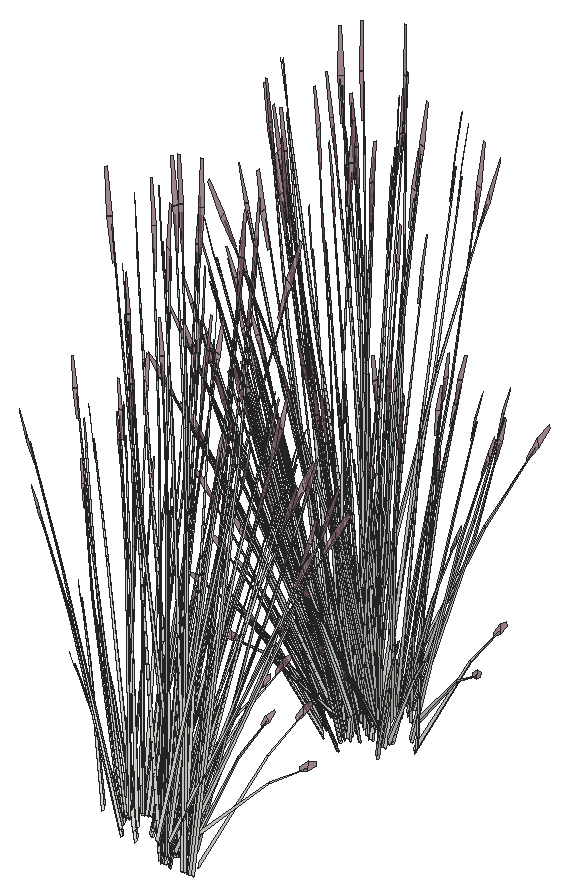
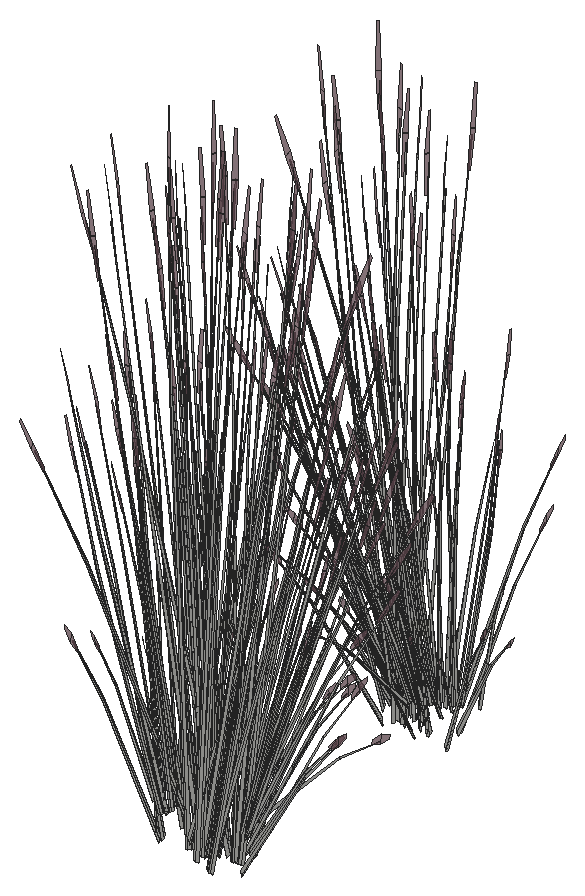
# SketchUp Ruby script. Lengths in inches.
U = 1.inch
M = Sketchup.active_model
def pt(a) = Geom::Point3d.new(a.map { |v| v * U })
def face(e, loops, mat)
  f = e.add_face(loops[0].map { |a| pt(a) })
  loops[1..].each { |l| e.add_face(l.map { |a| pt(a) }).erase! }
  f.material = f.back_material = mat if mat
  f
end
# faces: each face lists its corners as indices into pts; further lists are holes
def faces(e, pts, list, mat = nil) = list.each { |f| face(e, (f[0].is_a?(Array) ? f : [f]).map { |l| l.map { |i| pts[i] } }, mat) }
# xy, xz, yz: faces in a plane at the given z, y or x. An outline is a flat list of corners, or four numbers for a rectangle; further outlines are holes
def ring(l) = l.size == 4 ? [[l[0], l[1]], [l[2], l[1]], [l[2], l[3]], [l[0], l[3]]] : l.each_slice(2).to_a
def flat(e, list, mat, &to3) = list.each { |f| face(e, (f[0].is_a?(Array) ? f : [f]).map { |l| ring(l).map { |u, v| to3.(u, v) } }, mat) }
def xy(e, z, list, mat = nil) = flat(e, list, mat) { |x, y| [x, y, z] }
def xz(e, y, list, mat = nil) = flat(e, list, mat) { |x, z| [x, y, z] }
def yz(e, x, list, mat = nil) = flat(e, list, mat) { |y, z| [x, y, z] }
def lines(e, pts, list) = list.each { |a, b| e.add_line(pt(pts[a]), pt(pts[b])) }
# prism: a flat outline (further loops are holes) pulled along v
def prism(e, loops, v, mat = nil)
  f = face(e, loops, mat); d = Geom::Vector3d.new(v.map { |x| x * U })
  f.pushpull(f.normal.samedirection?(d) ? d.length : -d.length)
end
def box(e, o, s, mat = nil) = prism(e, [[o, [o[0] + s[0], o[1], o[2]], [o[0] + s[0], o[1] + s[1], o[2]], [o[0], o[1] + s[1], o[2]]]], [0, 0, s[2]], mat)
def at(x, y, z, deg = 0) = Geom::Transformation.translation(pt([x, y, z])) * Geom::Transformation.rotation(ORIGIN, Z_AXIS, deg.degrees)
def axes(o, x, y, z) = Geom::Transformation.new([*x, 0, *y, 0, *z, 0, *pt(o).to_a, 1])
def part(name) = M.definitions.add(name)
# library, detail: a bought-in or finely detailed component or shape, given as its bounding box
def library(name, o, s) = part(name).tap { |d| box(d.entities, o, s) }
def detail(e, o, s) = box(e.add_group.entities, o, s)
def put(e, d, t, mat = nil) = e.add_instance(d, t).tap { |i| i.material = mat if mat }
def group(e, t, mat = nil) = e.add_group.tap { |g| g.transformation = t; g.material = mat if mat }.entities
root = M.entities
M.materials.add("LightPink_Translucent").color = [144, 107, 117]
M.materials["LightPink_Translucent"].alpha = 0.75
c1 = part("blade")
p = [[2.15,0.21,22],[0,0.17,0],[0.09,0.45,0],[2.18,0.31,22],[2.29,0.31,22],[0.38,0.45,0],
  [2.48,0.24,33],[2.49,0.24,33],[2.48,0.22,33]]
faces(c1.entities,p,[[0,1,2,3],[4,5,2,3],[6,3,4,7],[8,0,3,6]])
c2 = part("seeds")
p = [[0.3,-0.1,1.38],[-0.01,-0.03,1.59],[-0.01,-0.03,0.03],[0.14,-0.07,-0.07],[0.29,-0.03,3],[0.15,0.01,3.11]]
faces(c2.entities,p,[[0,1,2,3],[1,0,4,5]],"LightPink_Translucent")
c3 = part("blade with seeds")
put(c3.entities,c1,at(0,0,0))
put(c3.entities,c2,axes([2.4,0.25,30.99],[1.5799,-0.05474,1.17369],[-0.12525,1.92788,0.29478],[-0.07173,-0.02425,1.56792]))
put(root,c3,axes([359.76,228.125,201.54],[0.11943,-0.00833,1.31208],[0.32759,-0.38275,-0.2075],[0.21244,0.05052,0.10523]))
put(root,c3,axes([358.36,228.87,199.64],[-0.34375,-0.4954,-0.03857],[0.58235,-0.27531,0.38706],[-0.1435,0.04717,1.22723]))
put(root,c3,axes([358.24,227.67,199.96],[0.41131,0.296,0.1086],[-0.34309,0.33395,-0.3101],[-0.0955,0.04515,0.95058]))
put(root,c3,axes([354.99,227.75,201.55],[-0.13808,-0.45342,0.36002],[0.54163,-0.07869,0.29685],[-0.15963,0.10664,0.74497]))
put(root,c3,axes([354.88,227.66,201.55],[-0.3822,-0.20719,0.04823],[0.22252,-0.29505,0.37966],[-0.12254,0.09539,0.57892]))
put(root,c3,axes([355.06,227.12,200.91],[0.19317,-0.10421,1.28532],[0.16263,0.48153,0.10393],[-0.30326,0.10883,0.54946]))
put(root,c3,axes([359.3,228.1875,201.74],[0.55654,0.01186,-0.53284],[-0.03738,0.49951,0.0643],[0.23578,0.05271,0.75375]))
put(root,c3,axes([358.67,228.59,199.86],[0.52105,-0.24633,0.37238],[0.31144,0.44171,0],[-0.11867,0.0561,1.18128]))
put(root,c3,axes([357.93,228.2,199.72],[0.24206,0.56598,-0.04509],[-0.69162,0.19832,0],[0.00845,0.01976,1.2913]))
put(root,c3,axes([358.2,228.81,199.52],[-0.51941,-0.1219,-0.23233],[0.13078,-0.42928,0.23233],[-0.10471,0.0495,1.0423]))
put(root,c3,axes([354.45,227.9375,199.94],[0.19348,0.04044,1.07251],[0.1247,0.41309,-0.23066],[-0.26282,0.07733,0.45856]))
put(root,c3,axes([355.32,227.6,201.79],[0.48462,-0.07041,0.2656],[0.12797,0.4025,-0.3429],[-0.13888,0.10811,0.65611]))
put(root,c3,axes([360.21,227.17,199.78],[0.69617,0,0],[0,0.55062,-0.38706],[0,0.12541,1.22783]))
put(root,c3,axes([353.46,227.42,201.53],[0.07105,0.01321,1.33037],[0.2198,0.43529,-0.12571],[-0.14545,0.11425,0.23543]))
put(root,c3,axes([359.93,227.46,199.65],[-0.69582,-0.00394,-0.03732],[0,-0.55062,0.37457],[-0.02187,0.12535,1.18764]))
put(root,c3,axes([358.43,226.98,200],[0.62699,0.23507,-0.21822],[-0.3019,0.49615,-0.37502],[0.0197,0.12182,1.19781]))
put(root,c3,axes([354.05,228.8,200.07],[0.23202,-0.22328,0.86145],[0.09155,0.35348,0.63294],[-0.16768,0.06329,0.18974]))
put(root,c3,axes([359.64,228.39,201.39],[0.31678,0.30846,-0.2656],[-0.36171,0.29199,0.3429],[0.18378,0.04443,0.65611]))
put(root,c3,axes([359.79,227.54,199.52],[-0.38863,0.30738,-0.23233],[-0.38863,-0.30738,0.23233],[0,0.09901,1.0423]))
put(root,c3,axes([358.11,227.57,200],[0.06488,0.56215,-0.21822],[-0.6757,0.03399,-0.37502],[-0.11898,0.07488,1.19781]))
put(root,c3,axes([359.47,228.51,201.55],[-0.02803,0.37463,0.04823],[-0.42332,-0.01027,0.37966],[0.16216,0.0392,0.57892]))
put(root,c3,axes([358.36,227.35,199.66],[-0.27012,0.44393,-0.33554],[-0.56127,-0.21365,0.16149],[0,0.10233,1.07733]))
put(root,c3,axes([354.93,227.84,201.39],[-0.48462,0.07041,-0.2656],[-0.12797,-0.4025,0.3429],[-0.13888,0.10811,0.65611]))
put(root,c3,axes([359.51,228.39,201.55],[-0.41051,0.32462,0.36002],[-0.35404,-0.34474,0.29685],[0.1926,0.05988,0.74497]))
put(root,c3,axes([354.22,228.74,202.23],[0.49129,0.13151,-0.04866],[-0.15113,0.40475,-0.22062],[-0.08035,0.06145,0.72768]))
put(root,c3,axes([357.71,227.99,199.54],[-0.375,0.3703,-0.46765],[-0.46584,-0.33578,-0.12274],[-0.15027,0.09237,1.03225]))
put(root,c3,axes([358.21,228.77,201.79],[-0.08599,-0.39682,0.2656],[0.49155,-0.10478,-0.3429],[0.13203,0.11372,0.65611]))
put(root,c3,axes([358.375,228.62,199.75],[0.697,0.16013,0.23067],[-0.17437,0.57237,-0.27369],[-0.11536,0.07164,1.23664]))
put(root,c3,axes([358.32,229,199.51],[-0.52105,0.24633,-0.37238],[-0.31144,-0.44171,0],[-0.11867,0.0561,1.18128]))
put(root,c3,axes([360.06,227.55,199.51],[0,0.49266,-0.37238],[-0.62289,0,0],[0,0.11221,1.18128]))
put(root,c3,axes([358.5,227.6,200.91],[-0.2068,-0.08488,1.28532],[0.42797,-0.35609,0.10393],[0.26673,0.16064,0.54946]))
put(root,c3,axes([358.54,226.48,201.36],[-0.48108,-0.25598,1.03712],[0.50798,-0.39855,0.44749],[0.15521,0.24018,1.00248]))
put(root,c3,axes([355.07,227.5625,201.78],[0.515,0.27165,-0.0912],[-0.2967,0.3934,-0.50621],[-0.1455,0.13675,0.76918]))
put(root,c3,axes([359.26,228.57,200.07],[-0.31347,-0.14166,0.86145],[0.40476,-0.14393,0.63294],[0.10917,0.12192,0.18974]))
put(root,c3,axes([358.16,228.97,201.78],[0.33176,-0.4217,-0.0912],[0.48044,0.24295,-0.50621],[0.16701,0.11914,0.76918]))
put(root,c3,axes([355.76,227.44,200.91],[0.13906,-0.15138,1.28532],[0.35111,0.40859,0.10393],[-0.24082,0.18608,0.54946]))
put(root,c3,axes([355.33,227.89,201.51],[0.14302,0.44985,-0.38324],[-0.54163,0.07869,-0.29685],[-0.15522,0.12083,0.7333]))
put(root,c3,axes([355.98,228.4,201.79],[0.3767,-0.25939,0.2656],[0.3566,0.29618,-0.3429],[-0.05426,0.15048,0.65611]))
put(root,c3,axes([358.8,228.93,199.78],[0.34808,0.49367,0],[-0.58235,0.27531,-0.38706],[-0.13264,0.0627,1.22783]))
put(root,c3,axes([357.73,229.32,201.53],[0.00165,-0.05965,1.33037],[0.47711,-0.26315,-0.12571],[0.16572,0.09393,0.23543]))
put(root,c3,axes([359.35,229.09,199.12],[0.04056,-0.07113,1.32257],[0.51066,-0.20948,-0.20205],[0.15482,0.10842,0.22528]))
put(root,c3,axes([358.5,226.97,200.13],[-0.01521,-0.46386,1.05954],[0.68831,0.12024,0.44862],[-0.1628,0.25382,1.00012]))
put(root,c3,axes([358.68,227.48,199.57],[0.20414,0.45107,-0.51909],[-0.58805,0.16245,-0.13624],[0.02256,0.15274,1.1458]))
put(root,c3,axes([355.63,228.64,201.55],[-0.45752,-0.02296,0.04823],[0.01254,-0.34663,0.37966],[-0.04787,0.13278,0.57892]))
put(root,c3,axes([354.66,229.03,199.12],[0.07468,0.04922,1.32257],[0.12663,0.45605,-0.20205],[-0.16551,0.09725,0.22528]))
put(root,c3,axes([355.78,228.67,201.55],[-0.39645,-0.33614,0.36002],[0.42102,-0.2899,0.29685],[-0.07313,0.15771,0.74497]))
put(root,c3,axes([358.56,228.76,201.51],[0.54938,-0.11711,-0.38324],[0.0961,0.44351,-0.29685],[0.14756,0.1271,0.7333]))
put(root,c3,axes([357.03,228.83,201.79],[0.16784,-0.37886,0.2656],[0.48968,0.1105,-0.3429],[0.0449,0.15254,0.65611]))
put(root,c3,axes([359.3125,229.21,200],[-0.35702,-0.01545,0.78795],[0.23577,-0.32816,0.43504],[0.14104,0.11659,0.61808]))
put(root,c3,axes([358.29,229.125,201.55],[-0.25304,0.31296,0.04823],[-0.36033,-0.18221,0.37966],[0.11649,0.10034,0.57892]))
put(root,c3,axes([357.69,230.18,202.23],[0.38473,-0.28263,-0.04866],[0.35252,0.30954,-0.22062],[0.02482,0.08771,0.72768]))
put(root,c3,axes([358.39,229.04,201.55],[-0.55374,0.11306,0.36002],[-0.0961,-0.44351,0.29685],[0.13023,0.13071,0.74497]))
put(root,c3,axes([355.66,227.82,200.91],[0.10366,-0.16934,1.28532],[0.43488,0.35044,0.10393],[-0.19618,0.21841,0.54946]))
put(root,c3,axes([358.15,228.42,199.94],[0.00982,-0.16331,1.07251],[0.4695,-0.18242,-0.23066],[0.14493,0.19547,0.45856]))
put(root,c3,axes([356.88,229.17,201.55],[-0.41024,0.16744,0.04823],[-0.2008,-0.30532,0.37966],[0.03962,0.13459,0.57892]))
put(root,c3,axes([355.78,228.77,201.39],[-0.3767,0.25939,-0.2656],[-0.3566,-0.29618,0.3429],[-0.05426,0.15048,0.65611]))
put(root,c3,axes([354.48,228.69,201.54],[-0.01384,0.09749,1.31208],[0.39274,0.33916,-0.2075],[-0.10282,0.16039,0.10523]))
put(root,c3,axes([355.74,228.47,202.05],[0.61188,0.02441,-0.10123],[-0.01672,0.46217,-0.56189],[-0.0425,0.178,0.85379]))
put(root,c3,axes([356.87,228.99,201.78],[0.54481,-0.22937,-0.0912],[0.26773,0.4071,-0.50621],[0.07188,0.17155,0.76918]))
put(root,c3,axes([357.03,229.14,201.8],[-0.54859,-0.1288,0.39962],[0.18759,-0.42344,0.32951],[0.03297,0.16652,0.82692]))
put(root,c3,axes([356.02,229.78,200.07],[-0.01441,-0.29294,0.86145],[0.36003,0.20894,0.63294],[-0.07081,0.13963,0.18974]))
put(root,c3,axes([356.97,229.08,199.12],[0.0901,-0.02681,1.32257],[0.54199,0.14755,-0.20205],[0.01585,0.1663,0.22528]))
put(root,c3,axes([356.15,228.65,201.75],[0.39855,0.33102,-0.4254],[-0.42102,0.2899,-0.32951],[-0.06064,0.16819,0.81396]))
put(root,c3,axes([355.72,229.15,200.12],[0.50577,-0.08724,0.04881],[0.11627,0.35148,-0.64728],[-0.03206,0.17792,0.5802]))
put(root,c3,axes([357.34,228.97,201.51],[0.54728,0.1235,-0.38324],[-0.18759,0.42344,-0.29685],[0.05018,0.17048,0.7333]))
put(root,c3,axes([357.65,228.1,200.91],[-0.12726,-0.15818,1.28532],[0.58807,-0.13317,0.10393],[0.13291,0.24832,0.54946]))
put(root,c3,axes([357.09,229.23,201.39],[-0.16784,0.37886,-0.2656],[-0.48968,-0.1105,0.3429],[0.0449,0.15254,0.65611]))
put(root,c3,axes([356.03,228.5,202],[-0.01449,0.45571,-0.59145],[-0.61002,-0.03061,0.07138],[-0.06438,0.19306,0.83667]))
put(root,c3,axes([354.4375,229.69,201.53],[0.06316,-0.02974,1.33037],[0.52204,0.19785,-0.12571],[-0.01227,0.16473,0.23543]))
put(root,c3,axes([356.61,228.17,200.91],[-0.01363,-0.18909,1.28532],[0.5906,0.12544,0.10393],[-0.03653,0.26947,0.54946]))
put(root,c3,axes([357.14,228.89,201.74],[0.26572,0.40059,-0.53284],[-0.54698,0.22325,0.0643],[0.06214,0.19355,0.75375]))
put(root,c3,axes([355.6,229.52,199.94],[0.17569,-0.07772,1.07251],[0.43377,0.23434,-0.23066],[-0.12911,0.20277,0.45856]))
put(root,c3,axes([356.74,229.9,201.54],[0.07057,0.07933,1.31208],[0.56952,0.03117,-0.2075],[0.05727,0.17496,0.10523]))
put(root,c3,axes([355.83,229.14,200.52],[0.01223,-0.25433,1.15759],[0.55017,0.13434,0.15997],[-0.04767,0.27105,0.54661]))
put(root,c3,axes([356.25,245.91,200.91],[0.12726,0.15818,1.28532],[-0.58807,0.13317,0.10393],[-0.13291,-0.24832,0.54946]))
put(root,c3,axes([357.22,244.86,201.54],[-0.08515,-0.06907,1.31208],[-0.56828,0.04379,-0.2075],[-0.0907,-0.16522,0.10523]))
put(root,c3,axes([358.54,245.68,199.94],[-0.15825,0.09972,1.07251],[-0.47395,-0.17454,-0.23066],[0.08785,-0.21706,0.45856]))
put(root,c3,axes([357.82,246.03,201.74],[-0.26572,-0.40059,-0.53284],[0.54698,-0.22325,0.0643],[-0.06214,-0.19355,0.75375]))
put(root,c3,axes([356.09,245.49,199.94],[-0.03371,0.16116,1.07251],[-0.49286,0.13491,-0.23066],[-0.11521,-0.20831,0.45856]))
put(root,c3,axes([357.36,245.14,199.12],[-0.09338,0.01775,1.32257],[-0.51641,-0.1998,-0.20205],[0.00867,-0.16666,0.22528]))
put(root,c3,axes([358.92,246.42,201.74],[0.01449,-0.45571,-0.53284],[0.61002,0.03061,0.0643],[0.06438,-0.19306,0.75375]))
put(root,c3,axes([359.77,245.71,201.54],[-0.00537,-0.09805,1.31208],[-0.45391,-0.28338,-0.2075],[0.07018,-0.17178,0.10523]))
put(root,c3,axes([357.87,245.69,201.39],[0.16784,-0.37886,-0.2656],[0.48968,0.1105,0.3429],[-0.0449,-0.15254,0.65611]))
put(root,c3,axes([358.24,246.19,200.91],[-0.10366,0.16934,1.28532],[-0.43488,-0.35044,0.10393],[0.19618,-0.21841,0.54946]))
put(root,c3,axes([359.65,245.36,201.53],[-0.05654,0.03763,1.33037],[-0.55396,-0.12696,-0.12571],[-0.02005,-0.16422,0.23543]))
put(root,c3,axes([357.62,245.95,201.51],[-0.54728,-0.1235,-0.38324],[0.18759,-0.42344,-0.29685],[-0.05018,-0.17048,0.7333]))
put(root,c3,axes([357.95,244.89,200.07],[0.07142,0.28728,0.86145],[-0.3962,-0.15911,0.63294],[0.04263,-0.1471,0.18974]))
put(root,c3,axes([358.8,246.27,201.51],[-0.39855,-0.33102,-0.38324],[0.42102,-0.2899,-0.29685],[0.06064,-0.16819,0.7333]))
put(root,c3,axes([356.64,244.64,201.53],[-0.01039,0.05905,1.33037],[-0.51226,0.21431,-0.12571],[-0.15074,-0.10955,0.23543]))
put(root,c3,axes([356.52,245.69,201.82],[0.62019,-0.12663,0.40322],[0.10763,0.49673,0.33247],[-0.14586,-0.1464,0.83437]))
put(root,c3,axes([357.93,245.78,201.55],[0.54859,0.1288,0.36002],[-0.18759,0.42344,0.29685],[-0.03297,-0.16652,0.74497]))
put(root,c3,axes([358.08,245.93,201.78],[-0.54481,0.22937,-0.0912],[-0.26773,-0.4071,-0.50621],[-0.07188,-0.17155,0.76918]))
put(root,c3,axes([359.22,246.44,201.78],[-0.61188,-0.02441,-0.0912],[0.01672,-0.46217,-0.50621],[0.0425,-0.178,0.76918]))
put(root,c3,axes([359.17,246.15,201.39],[0.3767,-0.25939,-0.2656],[0.3566,0.29618,0.3429],[0.05426,-0.15048,0.65611]))
put(root,c3,axes([355.92,245.23,200.07],[0.29042,0.17147,0.86145],[-0.42295,0.10307,0.63294],[-0.0905,-0.13178,0.18974]))
put(root,c3,axes([358.07,245.75,201.55],[0.41024,-0.16744,0.04823],[0.2008,0.30532,0.37966],[-0.03962,-0.13459,0.57892]))
put(root,c3,axes([356.62,246.14,201.74],[-0.47473,-0.23813,-0.53284],[0.33738,-0.41728,0.0643],[-0.172,-0.14218,0.75375]))
put(root,c3,axes([356.45,245.83,201.39],[-0.08599,-0.39682,-0.2656],[0.49155,-0.10478,0.3429],[-0.13203,-0.11372,0.65611]))
put(root,c3,axes([356.67,245.79,201.55],[0.25304,-0.31296,0.04823],[0.36033,0.18221,0.37966],[-0.11649,-0.10034,0.57892]))
put(root,c3,axes([355.6875,245.75,199.12],[-0.05393,0.0649,1.32257],[-0.545,0.13993,-0.20205],[-0.13166,-0.12729,0.22528]))
put(root,c3,axes([356.59,247.54,199.57],[-0.22864,-0.5052,-0.52377],[0.65862,-0.18195,-0.13747],[-0.02527,-0.17107,1.15612]))
put(root,c3,axes([355.4,246.41,200.91],[0.2068,0.08488,1.28532],[-0.42797,0.35609,0.10393],[-0.26673,-0.16064,0.54946]))
put(root,c3,axes([359.64,245.99,199.12],[-0.08333,-0.03881,1.32257],[-0.21404,-0.4336,-0.20205],[0.14439,-0.11767,0.22528]))
put(root,c3,axes([357.92,246.09,201.79],[-0.16784,0.37886,0.2656],[-0.48968,-0.1105,-0.3429],[-0.0449,-0.15254,0.65611]))
put(root,c3,axes([356.4,246.16,201.51],[-0.54938,0.11711,-0.38324],[-0.0961,-0.44351,-0.29685],[-0.14756,-0.1271,0.7333]))
put(root,c3,axes([359.17,246.25,201.55],[0.39645,0.33614,0.36002],[-0.42102,0.2899,0.29685],[0.07313,-0.15771,0.74497]))
put(root,c3,axes([356.78,245.76,202.07],[-0.37157,0.4723,-0.10215],[-0.5381,-0.2721,-0.56695],[-0.18705,-0.13344,0.86148]))
put(root,c3,axes([359.32,246.28,201.55],[0.45752,0.02296,0.04823],[-0.01254,0.34663,0.37966],[0.04787,-0.13278,0.57892]))
put(root,c3,axes([358.98,246.52,201.79],[-0.3767,0.25939,0.2656],[-0.3566,-0.29618,-0.3429],[0.05426,-0.15048,0.65611]))
put(root,c3,axes([359.64,247.21,201.74],[0.29081,-0.38873,-0.53284],[0.5096,0.27626,0.0643],[0.17364,-0.14084,0.75375]))
put(root,c3,axes([356.5,246.08,199.78],[-0.34808,-0.49367,0],[0.58235,-0.27531,-0.38706],[0.13264,-0.0627,1.22783]))
put(root,c3,axes([359.625,247.03,201.51],[-0.14302,-0.44985,-0.38324],[0.54163,-0.07869,-0.29685],[0.15522,-0.12083,0.7333]))
put(root,c3,axes([357.26,245.49,199.6],[-0.38473,0.28263,-0.02919],[-0.35252,-0.30954,-0.13237],[-0.02482,-0.08771,0.43661]))
put(root,c3,axes([355.36,245.625,201.54],[-0.11979,-0.00348,1.31208],[-0.38137,0.34775,-0.2075],[-0.20349,-0.07106,0.10523]))
put(root,c3,axes([359.88,247.35,201.78],[-0.515,-0.27165,-0.0912],[0.2967,-0.3934,-0.50621],[0.1455,-0.13675,0.76918]))
put(root,c3,axes([357.75,248.84,200.49],[0.48111,0.19866,1.13446],[-0.47133,0.42798,0.44862],[-0.21112,-0.25366,0.95105]))
put(root,c3,axes([356.75,246.15,201.79],[0.08599,0.39682,0.2656],[-0.49155,0.10478,-0.3429],[-0.13203,-0.11372,0.65611]))
put(root,c3,axes([355.24,247.46,199.51],[0,-0.49266,-0.37238],[0.62289,0,0],[0,-0.11221,1.18128]))
put(root,c3,axes([356.97,246.01,199.51],[0.52105,-0.24633,-0.37238],[0.31144,0.44171,0],[0.11867,-0.0561,1.18128]))
put(root,c3,axes([360.0625,246.86,199.94],[-0.19889,-0.01459,1.07251],[-0.20376,-0.39145,-0.23066],[0.24434,-0.11074,0.45856]))
put(root,c3,axes([355.27,246.41,201.82],[0.45978,-0.36358,0.40322],[0.39653,0.38611,0.33247],[-0.21571,-0.06707,0.83437]))
put(root,c3,axes([361.15,247.24,201.53],[-0.07272,-0.00374,1.33037],[-0.30197,-0.40092,-0.12571],[0.12127,-0.13182,0.23543]))
put(root,c3,axes([357.59,247.02,199.54],[0.375,-0.3703,-0.46765],[0.46584,0.33578,-0.12274],[0.15027,-0.09237,1.03225]))
put(root,c3,axes([360.29,246.14,200.07],[-0.18544,0.25079,0.86145],[-0.15939,-0.33694,0.63294],[0.15316,-0.08443,0.18974]))
put(root,c3,axes([360.03,247.08,201.39],[0.48462,-0.07041,-0.2656],[0.12797,0.4025,0.3429],[0.13888,-0.10811,0.65611]))
put(root,c3,axes([355.48,246.41,201.55],[0.02803,-0.37463,0.04823],[0.42332,0.01027,0.37966],[-0.16216,-0.0392,0.57892]))
put(root,c3,axes([356.93,247.67,199.66],[0.27012,-0.44393,-0.33554],[0.56127,0.21365,0.16149],[0,-0.10233,1.07733]))
put(root,c3,axes([355.32,246.53,201.39],[-0.31678,-0.30846,-0.2656],[0.36171,-0.29199,0.3429],[-0.18378,-0.04443,0.65611]))
put(root,c3,axes([357.18,247.45,200],[-0.06488,-0.56215,-0.21822],[0.6757,-0.03399,-0.37502],[0.11898,-0.07488,1.19781]))
put(root,c3,axes([355.51,247.48,199.52],[0.38863,-0.30738,-0.23233],[0.38863,0.30738,0.23233],[0,-0.09901,1.0423]))
put(root,c3,axes([355.35,246,199.6],[-0.1606,0.40228,-0.02919],[-0.4943,-0.12375,-0.13237],[-0.07505,-0.0658,0.43661]))
put(root,c3,axes([359.63,247.32,201.79],[-0.48462,0.07041,0.2656],[-0.12797,-0.4025,-0.3429],[0.13888,-0.10811,0.65611]))
put(root,c3,axes([356.87,248.03,200],[-0.62699,-0.23507,-0.21822],[0.3019,-0.49615,-0.37502],[-0.0197,-0.12182,1.19781]))
put(root,c3,axes([355.08,247.84,199.78],[-0.69617,0,0],[0,-0.55062,-0.38706],[0,-0.12541,1.22783]))
put(root,c3,axes([355.2,246.85,199.94],[0.1087,0.13716,1.07251],[-0.25048,0.37284,-0.23066],[-0.25719,-0.08912,0.45856]))
put(root,c3,axes([357.09,246.2,199.52],[0.51941,0.1219,-0.23233],[-0.13078,0.42928,0.23233],[0.10471,-0.0495,1.0423]))
put(root,c3,axes([355.65,246.73,201.74],[-0.55654,-0.01186,-0.53284],[0.03738,-0.49951,0.0643],[-0.23578,-0.05271,0.75375]))
put(root,c3,axes([360.07,247.25,201.55],[0.3822,0.20719,0.04823],[-0.22252,0.29505,0.37966],[0.12254,-0.09539,0.57892]))
put(root,c3,axes([359.96,247.17,201.55],[0.13808,0.45342,0.36002],[-0.54163,0.07869,0.29685],[0.15963,-0.10664,0.74497]))
put(root,c3,axes([361.42,247.72,201.54],[0.07726,-0.07504,1.31208],[-0.09888,-0.46032,-0.2075],[0.19384,-0.08728,0.10523]))
put(root,c3,axes([355.625,247.69,199.75],[-0.51786,0.4142,0.23067],[-0.51817,-0.40984,-0.27369],[-0.01808,-0.11762,1.23664]))
put(root,c3,axes([354.9,245.92,201.53],[0.04127,0.04917,1.33037],[-0.19898,0.44196,-0.12571],[-0.20151,0.0032,0.23543]))
put(root,c3,axes([357.27,247.89,199.82],[0.6273,0.23878,0.18048],[-0.3019,0.49615,0.37502],[0,-0.11437,1.20407]))
put(root,c3,axes([357.03,248.56,199.83],[0.14756,-0.58378,-0.17572],[0.69966,0.10176,0.38453],[-0.12225,-0.08062,1.1733]))
put(root,c3,axes([355.47,246.83,201.51],[-0.40426,0.32635,-0.38324],[-0.35404,-0.34474,-0.29685],[-0.2054,-0.04965,0.7333]))
put(root,c3,axes([355.77,246.6875,201.79],[0.31678,0.30846,0.2656],[-0.36171,0.29199,-0.3429],[-0.18378,-0.04443,0.65611]))
put(root,c3,axes([354.56,247.27,200.07],[0.35544,-0.03525,0.86145],[-0.22547,0.31061,0.63294],[-0.17565,-0.04659,0.18974]))
put(root,c3,axes([357.07,247.55,200.04],[-0.60457,0.03041,0.33554],[-0.05467,-0.50484,-0.16149],[0.10823,-0.05117,1.07733]))
put(root,c3,axes([355.68,246.49,201.78],[-0.02981,0.50103,-0.0912],[-0.56442,-0.01369,-0.50621],[-0.21738,-0.0348,0.76918]))
put(root,c3,axes([355.51,247.92,199.86],[0,0.49266,0.37238],[-0.62289,0,0],[0,-0.11221,1.18128]))
put(root,c3,axes([359.9,248.41,201.78],[-0.28012,-0.44611,-0.0912],[0.49717,-0.21923,-0.50621],[0.20951,-0.05886,0.76918]))
put(root,c3,axes([359.88,248.03,201.51],[0.15083,-0.44814,-0.38324],[0.51712,0.15361,-0.29685],[0.2082,-0.04109,0.7333]))
put(root,c3,axes([359.0625,246.21,199.78],[0.34808,-0.49367,0],[0.58235,0.27531,-0.38706],[0.13264,0.0627,1.22783]))
put(root,c3,axes([354.96,247.18,200.91],[0.23093,-0.01116,1.28532],[-0.15319,0.4836,0.10393],[-0.32909,-0.02991,0.54946]))
put(root,c3,axes([356.98,248.32,199.66],[-0.33445,-0.41351,-0.33554],[0.50659,-0.29119,0.16149],[-0.10823,-0.05117,1.07733]))
put(root,c3,axes([357.05,247.74,199.77],[0.24206,0.5509,0.34316],[-0.69162,0.19157,0.13466],[0.00845,-0.10123,1.19142]))
put(root,c3,axes([360.43,248.16,199.49],[-0.35858,0.05912,1.06187],[-0.05708,-0.47061,0.06078],[0.25115,-0.07123,0.60425]))
put(root,c3,axes([361.08,247.74,199.7],[-0.34516,-0.31503,-0.04866],[0.37803,-0.28865,-0.22062],[0.10711,-0.02032,0.72768]))
put(root,c3,axes([356.92,248.17,200.04],[-0.27012,0.44393,0.33554],[-0.56127,-0.21365,-0.16149],[0,-0.10233,1.07733]))
put(root,c3,axes([357.92,247.78,199.65],[0,-0.57005,0],[0.69617,0,0],[0,0,1.34592]))
put(root,c3,axes([358.76,246.46,199.86],[-0.52105,-0.24633,0.37238],[0.31144,-0.44171,0],[0.11867,0.0561,1.18128]))
put(root,c3,axes([359.78,248.19,201.74],[0.48922,-0.21758,-0.53284],[0.27264,0.44789,0.0643],[0.23638,-0.05088,0.75375]))
put(root,c3,axes([356.68,248.48,199.54],[-0.57914,-0.08077,-0.46765],[0.12221,-0.49823,-0.12274],[-0.17283,-0.06037,1.03225]))
put(root,c3,axes([357.59,247.42,199.77],[-0.46162,0.4471,0.34316],[-0.54842,-0.39467,0.13466],[0.11129,-0.04462,1.19142]))
put(root,c3,axes([358.09,248.22,199.72],[-0.51786,-0.42404,-0.04598],[0.51817,-0.4243,0],[-0.01808,-0.01481,1.31678]))
put(root,c3,axes([356.79,246.6875,199.86],[-0.16083,0.48962,0.13232],[-0.58854,-0.13856,0.26315],[0.10167,-0.00238,1.20305]))
put(root,c3,axes([359.71,248.28,201.79],[-0.46269,-0.13744,0.2656],[0.13495,-0.40096,-0.3429],[0.18628,-0.03677,0.65611]))
put(root,c3,axes([354.86,247.55,201.55],[0.15729,-0.44921,0.36002],[0.51712,0.15361,0.29685],[-0.20336,0.027,0.74497]))
put(root,c3,axes([356.54,247.08,199.2],[-0.548,0.19724,0.96696],[-0.17442,-0.56594,0.37572],[0.3365,0.00941,1.09981]))
put(root,c3,axes([358.01,247.23,199.96],[0.1074,-0.43968,0.1086],[0.52474,0.07632,-0.3101],[0.0955,0.04515,0.95058]))
put(root,c3,axes([354.83,247.43,201.55],[-0.20448,-0.33592,0.04823],[0.37288,-0.16442,0.37966],[-0.16437,0.03244,0.57892]))
put(root,c3,axes([357.11,248.28,199.77],[0.70367,0.1038,0.34316],[-0.1432,0.58624,0.13466],[-0.10283,-0.05661,1.19142]))
put(root,c3,axes([360.82,247.85,199.12],[-0.0291,-0.0748,1.32257],[0.20181,-0.43752,-0.20205],[0.20357,-0.00629,0.22528]))
put(root,c3,axes([354.81,247.77,199.12],[0.01412,0.07764,1.32257],[-0.28464,0.40547,-0.20205],[-0.20218,-0.02044,0.22528]))
put(root,c3,axes([357.79,247.35,200.04],[-0.33445,-0.41351,0.33554],[0.50659,-0.29119,-0.16149],[0.10823,0.05117,1.07733]))
put(root,c3,axes([356.0625,249.24,199.52],[-0.13078,-0.42928,-0.23233],[0.51941,-0.1219,0.23233],[-0.10471,-0.0495,1.0423]))
put(root,c3,axes([356.73,249.21,199.86],[0.59825,-0.13076,0.13232],[0.14773,0.48663,0.26315],[-0.05336,-0.0709,1.20305]))
put(root,c3,axes([357.96,247.375,200],[0.56211,-0.32708,-0.21822],[0.3738,0.46216,-0.37502],[0.13869,0.04694,1.19781]))
put(root,c3,axes([360.2,248.24,201.39],[0.46269,0.13744,-0.2656],[-0.13495,0.40096,0.3429],[0.18628,-0.03677,0.65611]))
put(root,c3,axes([355.92,249.42,199.51],[-0.52105,-0.24633,-0.37238],[0.31144,-0.44171,0],[-0.11867,-0.0561,1.18128]))
put(root,c3,axes([359.38,246.5,199.51],[0.52105,0.24633,-0.37238],[-0.31144,0.44171,0],[0.11867,0.0561,1.18128]))
put(root,c3,axes([354.76,247.6,201.39],[-0.46269,-0.13744,-0.2656],[0.13495,-0.40096,0.3429],[-0.18628,0.03677,0.65611]))
put(root,c3,axes([358.39,247.91,199.65],[0.62289,0,0],[0,0.51004,0],[0,0,1.33805]))
put(root,c3,axes([357.33,248.55,200],[-0.56211,0.32708,-0.21822],[-0.3738,-0.46216,-0.37502],[-0.13869,-0.04694,1.19781]))
put(root,c3,axes([358.57,246.71,199.86],[-0.59825,0.13076,0.13232],[-0.14773,-0.48663,0.26315],[0.05336,0.0709,1.20305]))
put(root,c3,axes([358.93,247.74,200.91],[-0.23093,0.01116,1.28532],[0.15319,-0.4836,0.10393],[0.32909,0.02991,0.54946]))
